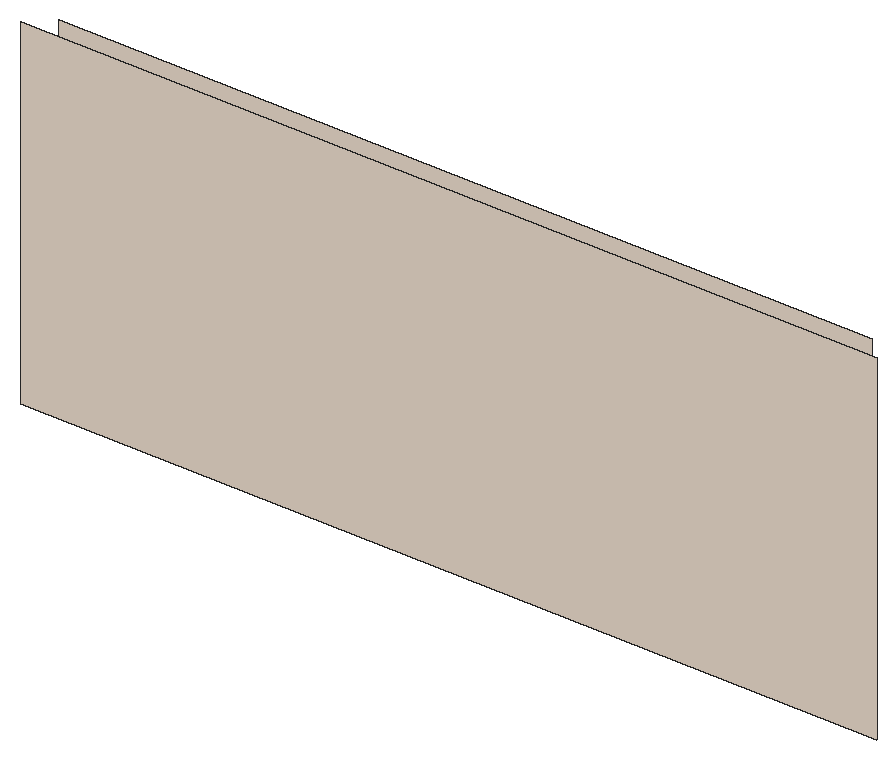
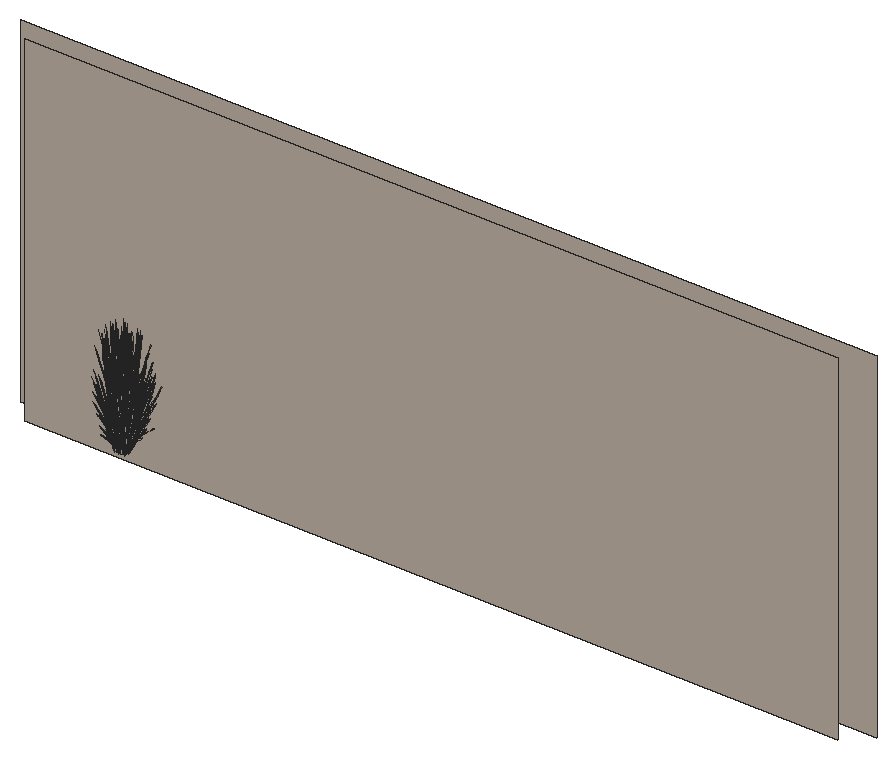
# SketchUp Ruby script. Lengths in inches.
U = 1.inch
M = Sketchup.active_model
def pt(a) = Geom::Point3d.new(a.map { |v| v * U })
def face(e, loops, mat)
  f = e.add_face(loops[0].map { |a| pt(a) })
  loops[1..].each { |l| e.add_face(l.map { |a| pt(a) }).erase! }
  f.material = f.back_material = mat if mat
  f
end
# faces: each face lists its corners as indices into pts; further lists are holes
def faces(e, pts, list, mat = nil) = list.each { |f| face(e, (f[0].is_a?(Array) ? f : [f]).map { |l| l.map { |i| pts[i] } }, mat) }
# xy, xz, yz: faces in a plane at the given z, y or x. An outline is a flat list of corners, or four numbers for a rectangle; further outlines are holes
def ring(l) = l.size == 4 ? [[l[0], l[1]], [l[2], l[1]], [l[2], l[3]], [l[0], l[3]]] : l.each_slice(2).to_a
def flat(e, list, mat, &to3) = list.each { |f| face(e, (f[0].is_a?(Array) ? f : [f]).map { |l| ring(l).map { |u, v| to3.(u, v) } }, mat) }
def xy(e, z, list, mat = nil) = flat(e, list, mat) { |x, y| [x, y, z] }
def xz(e, y, list, mat = nil) = flat(e, list, mat) { |x, z| [x, y, z] }
def yz(e, x, list, mat = nil) = flat(e, list, mat) { |y, z| [x, y, z] }
def lines(e, pts, list) = list.each { |a, b| e.add_line(pt(pts[a]), pt(pts[b])) }
# prism: a flat outline (further loops are holes) pulled along v
def prism(e, loops, v, mat = nil)
  f = face(e, loops, mat); d = Geom::Vector3d.new(v.map { |x| x * U })
  f.pushpull(f.normal.samedirection?(d) ? d.length : -d.length)
end
def box(e, o, s, mat = nil) = prism(e, [[o, [o[0] + s[0], o[1], o[2]], [o[0] + s[0], o[1] + s[1], o[2]], [o[0], o[1] + s[1], o[2]]]], [0, 0, s[2]], mat)
def at(x, y, z, deg = 0) = Geom::Transformation.translation(pt([x, y, z])) * Geom::Transformation.rotation(ORIGIN, Z_AXIS, deg.degrees)
def axes(o, x, y, z) = Geom::Transformation.new([*x, 0, *y, 0, *z, 0, *pt(o).to_a, 1])
def part(name) = M.definitions.add(name)
# library, detail: a bought-in or finely detailed component or shape, given as its bounding box
def library(name, o, s) = part(name).tap { |d| box(d.entities, o, s) }
def detail(e, o, s) = box(e.add_group.entities, o, s)
def put(e, d, t, mat = nil) = e.add_instance(d, t).tap { |i| i.material = mat if mat }
def group(e, t, mat = nil) = e.add_group.tap { |g| g.transformation = t; g.material = mat if mat }.entities
root = M.entities
M.materials.add("C01_Vanilla_Cream").color = [244, 228, 212]
M.materials.add("LightPink_Translucent").color = [144, 107, 117]
M.materials["LightPink_Translucent"].alpha = 0.75
c1 = part("blade")
p = [[2.15,0.21,22],[0,0.17,0],[0.09,0.45,0],[2.18,0.31,22],[2.29,0.31,22],[0.38,0.45,0],
  [2.48,0.24,33],[2.49,0.24,33],[2.48,0.22,33]]
faces(c1.entities,p,[[0,1,2,3],[4,5,2,3],[6,3,4,7],[8,0,3,6]])
c2 = part("seeds")
p = [[0.3,-0.1,1.38],[-0.01,-0.03,1.59],[-0.01,-0.03,0.03],[0.14,-0.07,-0.07],[0.29,-0.03,3],[0.15,0.01,3.11]]
faces(c2.entities,p,[[0,1,2,3],[1,0,4,5]],"LightPink_Translucent")
c3 = part("blade with seeds")
put(c3.entities,c1,at(0,0,0))
put(c3.entities,c2,axes([2.4,0.25,30.99],[1.5799,-0.05474,1.17369],[-0.12525,1.92788,0.29478],[-0.07173,-0.02425,1.56792]))
xz(root,0,[[0,300,360,444]],"C01_Vanilla_Cream")
xz(root,9,[[9,300,351,444]],"C01_Vanilla_Cream")
put(root,c3,axes([296.26,22.27,314.91],[0.23093,-0.01116,1.28532],[-0.15319,0.4836,0.10393],[-0.32909,-0.02991,0.54946]))
put(root,c3,axes([296.35,23.12,314.91],[0.19317,-0.10421,1.28532],[0.16263,0.48153,0.10393],[-0.30326,0.10883,0.54946]))
put(root,c3,axes([295.75,23.9375,313.94],[0.19348,0.04044,1.07251],[0.1247,0.41309,-0.23066],[-0.26282,0.07733,0.45856]))
put(root,c3,axes([297.46,22.62,314.51],[0.15825,-0.07127,1.32798],[0.05457,0.4976,0.10393],[-0.34278,0.06603,0.47463]))
put(root,c3,axes([295.76,22.95,315.54],[-0.09091,0.06396,1.31208],[0.00773,0.46734,-0.2075],[-0.20839,0.06078,0.10523]))
put(root,c3,axes([296.95,21.82,315.74],[-0.55654,-0.01186,-0.53284],[0.03738,-0.49951,0.0643],[-0.23578,-0.05271,0.75375]))
put(root,c3,axes([296.5,21.94,313.94],[0.1087,0.13716,1.07251],[-0.25048,0.37284,-0.23066],[-0.25719,-0.08912,0.45856]))
put(root,c3,axes([296.05,22.68,315.39],[-0.46269,-0.13744,-0.2656],[0.13495,-0.40096,0.3429],[-0.18628,0.03677,0.65611]))
put(root,c3,axes([296.69,21.49,314.91],[0.2068,0.08488,1.28532],[-0.42797,0.35609,0.10393],[-0.26673,-0.16064,0.54946]))
put(root,c3,axes([294.75,23.42,315.53],[0.07105,0.01321,1.33037],[0.2198,0.43529,-0.12571],[-0.14545,0.11425,0.23543]))
put(root,c3,axes([296.37,22.89,315.51],[-0.15083,0.44814,-0.38324],[-0.51712,-0.15361,-0.29685],[-0.2082,0.04109,0.7333]))
put(root,c3,axes([296.76,21.92,315.51],[-0.40426,0.32635,-0.38324],[-0.35404,-0.34474,-0.29685],[-0.2054,-0.04965,0.7333]))
put(root,c3,axes([296.11,22.86,313.12],[0.01412,0.07764,1.32257],[-0.28464,0.40547,-0.20205],[-0.20218,-0.02044,0.22528]))
put(root,c3,axes([296.19,21,315.53],[0.04127,0.04917,1.33037],[-0.19898,0.44196,-0.12571],[-0.20151,0.0032,0.23543]))
put(root,c3,axes([295.35,24.8,314.07],[0.23202,-0.22328,0.86145],[0.09155,0.35348,0.63294],[-0.16768,0.06329,0.18974]))
put(root,c3,axes([296.65,20.71,315.54],[-0.11979,-0.00348,1.31208],[-0.38137,0.34775,-0.2075],[-0.20349,-0.07106,0.10523]))
put(root,c3,axes([296.16,22.63,315.55],[0.15729,-0.44921,0.36002],[0.51712,0.15361,0.29685],[-0.20336,0.027,0.74497]))
put(root,c3,axes([296.35,22.5,315.78],[0.28012,0.44611,-0.0912],[-0.49717,0.21923,-0.50621],[-0.20951,0.05886,0.76918]))
put(root,c3,axes([296.98,21.58,315.78],[-0.02981,0.50103,-0.0912],[-0.56442,-0.01369,-0.50621],[-0.21738,-0.0348,0.76918]))
put(root,c3,axes([296.61,21.61,315.39],[-0.31678,-0.30846,-0.2656],[0.36171,-0.29199,0.3429],[-0.18378,-0.04443,0.65611]))
put(root,c3,axes([296.12,22.51,315.55],[-0.20448,-0.33592,0.04823],[0.37288,-0.16442,0.37966],[-0.16437,0.03244,0.57892]))
put(root,c3,axes([297.06,23.44,314.91],[0.13906,-0.15138,1.28532],[0.35111,0.40859,0.10393],[-0.24082,0.18608,0.54946]))
put(root,c3,axes([296.22,23.84,315.39],[-0.48462,0.07041,-0.2656],[-0.12797,-0.4025,0.3429],[-0.13888,0.10811,0.65611]))
put(root,c3,axes([295.96,25.03,313.12],[0.07468,0.04922,1.32257],[0.12663,0.45605,-0.20205],[-0.16551,0.09725,0.22528]))
put(root,c3,axes([295.85,22.35,314.07],[0.35544,-0.03525,0.86145],[-0.22547,0.31061,0.63294],[-0.17565,-0.04659,0.18974]))
put(root,c3,axes([296.29,23.75,315.55],[-0.13808,-0.45342,0.36002],[0.54163,-0.07869,0.29685],[-0.15963,0.10664,0.74497]))
put(root,c3,axes([296.57,21.5,315.82],[0.45978,-0.36358,0.40322],[0.39653,0.38611,0.33247],[-0.21571,-0.06707,0.83437]))
put(root,c3,axes([296.18,23.66,315.55],[-0.3822,-0.20719,0.04823],[0.22252,-0.29505,0.37966],[-0.12254,0.09539,0.57892]))
put(root,c3,axes([296.96,23.82,314.91],[0.10366,-0.16934,1.28532],[0.43488,0.35044,0.10393],[-0.19618,0.21841,0.54946]))
put(root,c3,axes([296.54,22.64,315.79],[0.46269,0.13744,0.2656],[-0.13495,0.40096,-0.3429],[-0.18628,0.03677,0.65611]))
put(root,c3,axes([296.62,23.89,315.51],[0.14302,0.44985,-0.38324],[-0.54163,0.07869,-0.29685],[-0.15522,0.12083,0.7333]))
put(root,c3,axes([296.78,21.49,315.55],[0.02803,-0.37463,0.04823],[0.42332,0.01027,0.37966],[-0.16216,-0.0392,0.57892]))
put(root,c3,axes([295.78,24.69,315.54],[-0.01384,0.09749,1.31208],[0.39274,0.33916,-0.2075],[-0.10282,0.16039,0.10523]))
put(root,c3,axes([297.97,23.5625,313.54],[-0.57914,-0.08077,-0.46765],[0.12221,-0.49823,-0.12274],[-0.17283,-0.06037,1.03225]))
put(root,c3,axes([298.08,20.85,316.07],[-0.37157,0.4723,-0.10215],[-0.5381,-0.2721,-0.56695],[-0.18705,-0.13344,0.86148]))
put(root,c3,axes([297.0625,21.77,315.79],[0.31678,0.30846,0.2656],[-0.36171,0.29199,-0.3429],[-0.18378,-0.04443,0.65611]))
put(root,c3,axes([297.92,21.23,315.74],[-0.47473,-0.23813,-0.53284],[0.33738,-0.41728,0.0643],[-0.172,-0.14218,0.75375]))
put(root,c3,axes([297.69,21.24,315.51],[-0.54938,0.11711,-0.38324],[-0.0961,-0.44351,-0.29685],[-0.14756,-0.1271,0.7333]))
put(root,c3,axes([297.21,24.51,313.51],[-0.52105,-0.24633,-0.37238],[0.31144,-0.44171,0],[-0.11867,-0.0561,1.18128]))
put(root,c3,axes([296.98,20.84,313.12],[-0.05393,0.0649,1.32257],[-0.545,0.13993,-0.20205],[-0.13166,-0.12729,0.22528]))
put(root,c3,axes([296.37,23.5625,315.78],[0.515,0.27165,-0.0912],[-0.2967,0.3934,-0.50621],[-0.1455,0.13675,0.76918]))
put(root,c3,axes([297.53,24.8,313.78],[-0.34808,0.49367,0],[-0.58235,-0.27531,-0.38706],[-0.13264,-0.0627,1.22783]))
put(root,c3,axes([295.52,24.74,316.23],[0.49129,0.13151,-0.04866],[-0.15113,0.40475,-0.22062],[-0.08035,0.06145,0.72768]))
put(root,c3,axes([296.62,23.6,315.79],[0.48462,-0.07041,0.2656],[0.12797,0.4025,-0.3429],[-0.13888,0.10811,0.65611]))
put(root,c3,axes([296.9,25.52,313.94],[0.17569,-0.07772,1.07251],[0.43377,0.23434,-0.23066],[-0.12911,0.20277,0.45856]))
put(root,c3,axes([296.65,21.09,313.6],[-0.1606,0.40228,-0.02919],[-0.4943,-0.12375,-0.13237],[-0.07505,-0.0658,0.43661]))
put(root,c3,axes([297.93,19.72,315.53],[-0.01039,0.05905,1.33037],[-0.51226,0.21431,-0.12571],[-0.15074,-0.10955,0.23543]))
put(root,c3,axes([297.38,20.58,313.94],[-0.03371,0.16116,1.07251],[-0.49286,0.13491,-0.23066],[-0.11521,-0.20831,0.45856]))
put(root,c3,axes([297.55,21,314.91],[0.12726,0.15818,1.28532],[-0.58807,0.13317,0.10393],[-0.13291,-0.24832,0.54946]))
put(root,c3,axes([298.63,23.64,314],[-0.56211,0.32708,-0.21822],[-0.3738,-0.46216,-0.37502],[-0.13869,-0.04694,1.19781]))
put(root,c3,axes([297.08,24.67,315.55],[-0.39645,-0.33614,0.36002],[0.42102,-0.2899,0.29685],[-0.07313,0.15771,0.74497]))
put(root,c3,axes([297.75,20.91,315.39],[-0.08599,-0.39682,-0.2656],[0.49155,-0.10478,0.3429],[-0.13203,-0.11372,0.65611]))
put(root,c3,axes([296.38,22.92,313.78],[-0.69617,0,0],[0,-0.55062,-0.38706],[0,-0.12541,1.22783]))
put(root,c3,axes([297.36,24.32,313.52],[-0.13078,-0.42928,-0.23233],[0.51941,-0.1219,0.23233],[-0.10471,-0.0495,1.0423]))
put(root,c3,axes([296.93,24.64,315.55],[-0.45752,-0.02296,0.04823],[0.01254,-0.34663,0.37966],[-0.04787,0.13278,0.57892]))
put(root,c3,axes([297.08,24.77,315.39],[-0.3767,0.25939,-0.2656],[-0.3566,-0.29618,0.3429],[-0.05426,0.15048,0.65611]))
put(root,c3,axes([299,23.99,313.54],[-0.375,0.3703,-0.46765],[-0.46584,-0.33578,-0.12274],[-0.15027,0.09237,1.03225]))
put(root,c3,axes([298.04,21.24,315.79],[0.08599,0.39682,0.2656],[-0.49155,0.10478,-0.3429],[-0.13203,-0.11372,0.65611]))
put(root,c3,axes([295.73,25.69,315.53],[0.06316,-0.02974,1.33037],[0.52204,0.19785,-0.12571],[-0.01227,0.16473,0.23543]))
put(root,c3,axes([296.92,22.78,313.75],[-0.51786,0.4142,0.23067],[-0.51817,-0.40984,-0.27369],[-0.01808,-0.11762,1.23664]))
put(root,c3,axes([299.05,23.92,314.49],[0.48111,0.19866,1.13446],[-0.47133,0.42798,0.44862],[-0.21112,-0.25366,0.95105]))
put(root,c3,axes([297.21,20.32,314.07],[0.29042,0.17147,0.86145],[-0.42295,0.10307,0.63294],[-0.0905,-0.13178,0.18974]))
put(root,c3,axes([299.26,23.79,313.85],[-0.54364,-0.39653,-0.18894],[0.45745,-0.44527,0.41347],[-0.14639,0.04639,1.26162]))
put(root,c3,axes([298.27,23.4,313.66],[-0.33445,-0.41351,-0.33554],[0.50659,-0.29119,0.16149],[-0.10823,-0.05117,1.07733]))
put(root,c3,axes([297.33,24.5,316],[-0.01449,0.45571,-0.59145],[-0.61002,-0.03061,0.07138],[-0.06438,0.19306,0.83667]))
put(root,c3,axes([297.32,25.78,314.07],[-0.01441,-0.29294,0.86145],[0.36003,0.20894,0.63294],[-0.07081,0.13963,0.18974]))
put(root,c3,axes([297.82,20.77,315.82],[0.62019,-0.12663,0.40322],[0.10763,0.49673,0.33247],[-0.14586,-0.1464,0.83437]))
put(root,c3,axes([298.99,23.7,313.66],[-0.60457,0.03041,-0.33554],[-0.05467,-0.50484,0.16149],[-0.10823,0.05117,1.07733]))
put(root,c3,axes([297.96,20.88,315.55],[0.25304,-0.31296,0.04823],[0.36033,0.18221,0.37966],[-0.11649,-0.10034,0.57892]))
put(root,c3,axes([297.83,24.55,313.86],[0.52105,0.24633,0.37238],[-0.31144,0.44171,0],[-0.11867,-0.0561,1.18128]))
put(root,c3,axes([297.12,25.14,314.52],[0.01223,-0.25433,1.15759],[0.55017,0.13434,0.15997],[-0.04767,0.27105,0.54661]))
put(root,c3,axes([298.32,23.64,313.83],[0.14756,-0.58378,-0.17572],[0.69966,0.10176,0.38453],[-0.12225,-0.08062,1.1733]))
put(root,c3,axes([298.58,23.78,313.96],[-0.1074,0.43968,0.1086],[-0.52474,-0.07632,-0.3101],[-0.0955,-0.04515,0.95058]))
put(root,c3,axes([298.52,19.95,315.54],[-0.08515,-0.06907,1.31208],[-0.56828,0.04379,-0.2075],[-0.0907,-0.16522,0.10523]))
put(root,c3,axes([299.62,25,313.51],[-0.52105,0.24633,-0.37238],[-0.31144,-0.44171,0],[-0.11867,0.0561,1.18128]))
put(root,c3,axes([296.54,22.55,313.51],[0,-0.49266,-0.37238],[0.62289,0,0],[0,-0.11221,1.18128]))
put(root,c3,axes([296.8,23.01,313.86],[0,0.49266,0.37238],[-0.62289,0,0],[0,-0.11221,1.18128]))
put(root,c3,axes([299.66,24.87,313.64],[-0.34375,-0.4954,-0.03857],[0.58235,-0.27531,0.38706],[-0.1435,0.04717,1.22723]))
put(root,c3,axes([297.45,24.65,315.75],[0.39855,0.33102,-0.4254],[-0.42102,0.2899,-0.32951],[-0.06064,0.16819,0.81396]))
put(root,c3,axes([299.5,24.81,313.52],[-0.51941,-0.1219,-0.23233],[0.13078,-0.42928,0.23233],[-0.10471,0.0495,1.0423]))
put(root,c3,axes([297.27,24.4,315.79],[0.3767,-0.25939,0.2656],[0.3566,0.29618,-0.3429],[-0.05426,0.15048,0.65611]))
put(root,c3,axes([298.16,23.12,314],[-0.62699,-0.23507,-0.21822],[0.3019,-0.49615,-0.37502],[-0.0197,-0.12182,1.19781]))
put(root,c3,axes([299.8,22.97,314.13],[-0.01521,-0.46386,1.05954],[0.68831,0.12024,0.44862],[-0.1628,0.25382,1.00012]))
put(root,c3,axes([297.03,24.47,316.05],[0.61188,0.02441,-0.10123],[-0.01672,0.46217,-0.56189],[-0.0425,0.178,0.85379]))
put(root,c3,axes([297.02,25.15,314.12],[0.50577,-0.08724,0.04881],[0.11627,0.35148,-0.64728],[-0.03206,0.17792,0.5802]))
put(root,c3,axes([299.41,23.57,314],[0.06488,0.56215,-0.21822],[-0.6757,0.03399,-0.37502],[-0.11898,0.07488,1.19781]))
put(root,c3,axes([297.88,22.62,313.57],[-0.22864,-0.5052,-0.52377],[0.65862,-0.18195,-0.13747],[-0.02527,-0.17107,1.15612]))
put(root,c3,axes([299.38,21.02,315.78],[-0.54481,0.22937,-0.0912],[-0.26773,-0.4071,-0.50621],[-0.07188,-0.17155,0.76918]))
put(root,c3,axes([298.91,21.04,315.51],[-0.54728,-0.1235,-0.38324],[0.18759,-0.42344,-0.29685],[-0.05018,-0.17048,0.7333]))
put(root,c3,axes([297.9,24.17,314.91],[-0.01363,-0.18909,1.28532],[0.5906,0.12544,0.10393],[-0.03653,0.26947,0.54946]))
put(root,c3,axes([296.8,22.5625,313.52],[0.38863,-0.30738,-0.23233],[0.38863,0.30738,0.23233],[0,-0.09901,1.0423]))
put(root,c3,axes([298.56,20.57,313.6],[-0.38473,0.28263,-0.02919],[-0.35252,-0.30954,-0.13237],[-0.02482,-0.08771,0.43661]))
put(root,c3,axes([298.4,23.36,313.77],[0.70367,0.1038,0.34316],[-0.1432,0.58624,0.13466],[-0.10283,-0.05661,1.19142]))
put(root,c3,axes([298.22,23.25,314.04],[-0.27012,0.44393,0.33554],[-0.56127,-0.21365,-0.16149],[0,-0.10233,1.07733]))
put(root,c3,axes([299.11,21.12,315.74],[-0.26572,-0.40059,-0.53284],[0.54698,-0.22325,0.0643],[-0.06214,-0.19355,0.75375]))
put(root,c3,axes([298.03,24.3,313.86],[0.59825,-0.13076,0.13232],[0.14773,0.48663,0.26315],[-0.05336,-0.0709,1.20305]))
put(root,c3,axes([298.8,24.375,313.65],[-0.56127,-0.22118,0],[0.27012,-0.45959,0],[0,0,1.2203]))
put(root,c3,axes([299.22,21.17,315.79],[-0.16784,0.37886,0.2656],[-0.48968,-0.1105,-0.3429],[-0.0449,-0.15254,0.65611]))
put(root,c3,axes([300.09,24.93,313.78],[0.34808,0.49367,0],[-0.58235,0.27531,-0.38706],[-0.13264,0.0627,1.22783]))
put(root,c3,axes([298.32,25.14,315.8],[-0.54859,-0.1288,0.39962],[0.18759,-0.42344,0.32951],[0.03297,0.16652,0.82692]))
put(root,c3,axes([298.18,25.17,315.55],[-0.41024,0.16744,0.04823],[-0.2008,-0.30532,0.37966],[0.03962,0.13459,0.57892]))
put(root,c3,axes([299.81,24.32,313.86],[0.16083,-0.48962,0.13232],[0.58854,0.13856,0.26315],[-0.10167,0.00238,1.20305]))
put(root,c3,axes([299.53,23.67,313.96],[0.41131,0.296,0.1086],[-0.34309,0.33395,-0.3101],[-0.0955,0.04515,0.95058]))
put(root,c3,axes([299.39,23.31,313.72],[-0.51786,-0.42404,-0.04598],[0.51817,-0.4243,0],[-0.01808,-0.01481,1.31678]))
put(root,c3,axes([299.52,23.46,314.04],[0.60457,-0.03041,0.33554],[0.05467,0.50484,-0.16149],[-0.10823,0.05117,1.07733]))
put(root,c3,axes([299.67,24.62,313.75],[0.697,0.16013,0.23067],[-0.17437,0.57237,-0.27369],[-0.11536,0.07164,1.23664]))
put(root,c3,axes([298.65,20.23,313.12],[-0.09338,0.01775,1.32257],[-0.51641,-0.1998,-0.20205],[0.00867,-0.16666,0.22528]))
put(root,c3,axes([299.97,24.59,313.86],[0.52105,-0.24633,0.37238],[0.31144,0.44171,0],[-0.11867,0.0561,1.18128]))
put(root,c3,axes([299.16,20.78,315.39],[0.16784,-0.37886,-0.2656],[0.48968,0.1105,0.3429],[-0.0449,-0.15254,0.65611]))
put(root,c3,axes([298.34,22.82,313.77],[0.24206,0.5509,0.34316],[-0.69162,0.19157,0.13466],[0.00845,-0.10123,1.19142]))
put(root,c3,axes([298.23,22.75,313.66],[0.27012,-0.44393,-0.33554],[0.56127,0.21365,0.16149],[0,-0.10233,1.07733]))
put(root,c3,axes([298.92,24.18,313.65],[-0.18165,-0.42474,0],[0.51872,-0.14874,0],[0,0,1.15778]))
put(root,c3,axes([298.26,25.08,313.12],[0.0901,-0.02681,1.32257],[0.54199,0.14755,-0.20205],[0.01585,0.1663,0.22528]))
put(root,c3,axes([298.38,25.23,315.39],[-0.16784,0.37886,-0.2656],[-0.48968,-0.1105,0.3429],[0.0449,0.15254,0.65611]))
put(root,c3,axes([299.66,23.35,313.66],[-0.27012,0.44393,-0.33554],[-0.56127,-0.21365,0.16149],[0,0.10233,1.07733]))
put(root,c3,axes([299.37,20.83,315.55],[0.41024,-0.16744,0.04823],[0.2008,0.30532,0.37966],[-0.03962,-0.13459,0.57892]))
put(root,c3,axes([298.04,25.9,315.54],[0.07057,0.07933,1.31208],[0.56952,0.03117,-0.2075],[0.05727,0.17496,0.10523]))
put(root,c3,axes([300.72,23.07,313.86],[-0.43742,-0.35886,0.13232],[0.44081,-0.34807,0.26315],[-0.04831,0.07329,1.20305]))
put(root,c3,axes([299.21,22.87,313.65],[0,-0.57005,0],[0.69617,0,0],[0,0,1.34592]))
put(root,c3,axes([299.22,20.86,315.55],[0.54859,0.1288,0.36002],[-0.18759,0.42344,0.29685],[-0.03297,-0.16652,0.74497]))
put(root,c3,axes([298.57,22.97,313.82],[0.6273,0.23878,0.18048],[-0.3019,0.49615,0.37502],[0,-0.11437,1.20407]))
put(root,c3,axes([299.5625,23.1,313.72],[0,0.56976,-0.04228],[-0.69617,0,0],[0,0.01791,1.34526]))
put(root,c3,axes([298.36,22.64,314.04],[-0.60457,0.03041,0.33554],[-0.05467,-0.50484,-0.16149],[0.10823,-0.05117,1.07733]))
put(root,c3,axes([298.33,24.83,315.79],[0.16784,-0.37886,0.2656],[0.48968,0.1105,-0.3429],[0.0449,0.15254,0.65611]))
put(root,c3,axes([298.08,21.77,313.86],[-0.16083,0.48962,0.13232],[-0.58854,-0.13856,0.26315],[0.10167,-0.00238,1.20305]))
put(root,c3,axes([299.23,24.2,313.72],[0.24206,0.56598,-0.04509],[-0.69162,0.19832,0],[0.00845,0.01976,1.2913]))
put(root,c3,axes([297.79,21.17,313.78],[-0.34808,-0.49367,0],[0.58235,-0.27531,-0.38706],[0.13264,-0.0627,1.22783]))
put(root,c3,axes([298.43,24.89,315.74],[0.26572,0.40059,-0.53284],[-0.54698,0.22325,0.0643],[0.06214,0.19355,0.75375]))
put(root,c3,axes([301.23,23.46,313.65],[-0.69582,-0.00394,-0.03732],[0,-0.55062,0.37457],[-0.02187,0.12535,1.18764]))
put(root,c3,axes([299.86,21.8,313.86],[-0.59825,0.13076,0.13232],[-0.14773,-0.48663,0.26315],[0.05336,0.0709,1.20305]))
put(root,c3,axes([299.25,19.98,314.07],[0.07142,0.28728,0.86145],[-0.3962,-0.15911,0.63294],[0.04263,-0.1471,0.18974]))
put(root,c3,axes([298.99,26.18,316.23],[0.38473,-0.28263,-0.04866],[0.35252,0.30954,-0.22062],[0.02482,0.08771,0.72768]))
put(root,c3,axes([298.88,22.51,313.77],[-0.46162,0.4471,0.34316],[-0.54842,-0.39467,0.13466],[0.11129,-0.04462,1.19142]))
put(root,c3,axes([299.67,23.21,313.66],[0.38863,0.31822,0],[-0.38863,0.31822,0],[0,0,1.2695]))
put(root,c3,axes([299.67,22.84,314.04],[0.27012,-0.44393,0.33554],[0.56127,0.21365,-0.16149],[0,0.10233,1.07733]))
put(root,c3,axes([299.43,24.38,313.65],[0.56127,0.22118,0],[-0.27012,0.45959,0],[0,0,1.31215]))
put(root,c3,axes([298.63,24.97,315.51],[0.54728,0.1235,-0.38324],[-0.18759,0.42344,-0.29685],[0.05018,0.17048,0.7333]))
put(root,c3,axes([298.16,24.99,315.78],[0.54481,-0.22937,-0.0912],[0.26773,0.4071,-0.50621],[0.07188,0.17155,0.76918]))
put(root,c3,axes([299.48,22.74,313.79],[-0.70367,-0.1038,0.36899],[0.1432,-0.58624,0.1448],[0.10283,0.05661,1.2811]))
put(root,c3,axes([300.95,20.44,315.53],[-0.05654,0.03763,1.33037],[-0.55396,-0.12696,-0.12571],[-0.02005,-0.16422,0.23543]))
put(root,c3,axes([300.51,21.53,315.78],[-0.61188,-0.02441,-0.0912],[0.01672,-0.46217,-0.50621],[0.0425,-0.178,0.76918]))
put(root,c3,axes([301.08,23.54,313.52],[-0.38863,0.30738,-0.23233],[-0.38863,-0.30738,0.23233],[0,0.09901,1.0423]))
put(root,c3,axes([299.97,23.48,313.57],[0.20414,0.45107,-0.51909],[-0.58805,0.16245,-0.13624],[0.02256,0.15274,1.1458]))
put(root,c3,axes([299.6875,23,313.65],[0.62289,0,0],[0,0.51004,0],[0,0,1.33805]))
put(root,c3,axes([300.27,21.6,315.79],[-0.3767,0.25939,0.2656],[-0.3566,-0.29618,-0.3429],[0.05426,-0.15048,0.65611]))
put(root,c3,axes([299.09,22.43,314.04],[-0.33445,-0.41351,0.33554],[0.50659,-0.29119,-0.16149],[0.10823,0.05117,1.07733]))
put(root,c3,axes([298.48,22.53,314],[-0.06488,-0.56215,-0.21822],[0.6757,-0.03399,-0.37502],[0.11898,-0.07488,1.19781]))
put(root,c3,axes([299.9,22.94,313.96],[0.51872,-0.14368,0.1086],[0.18165,0.41027,-0.3101],[0,0.09029,0.95058]))
put(root,c3,axes([300.1,21.36,315.51],[-0.39855,-0.33102,-0.38324],[0.42102,-0.2899,-0.29685],[0.06064,-0.16819,0.7333]))
put(root,c3,axes([299.72,22.98,314],[0.62699,0.23507,-0.21822],[-0.3019,0.49615,-0.37502],[0.0197,0.12182,1.19781]))
put(root,c3,axes([298.39,21.29,313.52],[0.51941,0.1219,-0.23233],[-0.13078,0.42928,0.23233],[0.10471,-0.0495,1.0423]))
put(root,c3,axes([299.83,20.77,313.94],[-0.15825,0.09972,1.07251],[-0.47395,-0.17454,-0.23066],[0.08785,-0.21706,0.45856]))
put(root,c3,axes([301.09,23.09,313.86],[0,-0.49266,0.37238],[0.62289,0,0],[0,0.11221,1.18128]))
put(root,c3,axes([301.35,23.55,313.51],[0,0.49266,-0.37238],[-0.62289,0,0],[0,0.11221,1.18128]))
put(root,c3,axes([299.6875,25.04,315.55],[-0.55374,0.11306,0.36002],[-0.0961,-0.44351,0.29685],[0.13023,0.13071,0.74497]))
put(root,c3,axes([298.27,21.09,313.51],[0.52105,-0.24633,-0.37238],[0.31144,0.44171,0],[0.11867,-0.0561,1.18128]))
put(root,c3,axes([299.58,25.125,315.55],[-0.25304,0.31296,0.04823],[-0.36033,-0.18221,0.37966],[0.11649,0.10034,0.57892]))
put(root,c3,axes([298.94,24.1,314.91],[-0.12726,-0.15818,1.28532],[0.58807,-0.13317,0.10393],[0.13291,0.24832,0.54946]))
put(root,c3,axes([299.3125,22.32,313.96],[0.1074,-0.43968,0.1086],[0.52474,0.07632,-0.3101],[0.0955,0.04515,0.95058]))
put(root,c3,axes([300.06,21.55,313.86],[-0.52105,-0.24633,0.37238],[0.31144,-0.44171,0],[0.11867,0.0561,1.18128]))
put(root,c3,axes([300.22,21.51,315.74],[0.01449,-0.45571,-0.53284],[0.61002,0.03061,0.0643],[0.06438,-0.19306,0.75375]))
put(root,c3,axes([299.6,24.125,313.64],[0.5845,-0.16716,-0.14398],[0.20539,0.48152,0.00006],[0.06452,-0.01848,1.30423]))
put(root,c3,axes([299.5,24.77,315.79],[-0.08599,-0.39682,0.2656],[0.49155,-0.10478,-0.3429],[0.13203,0.11372,0.65611]))
put(root,c3,axes([299.61,22.69,313.66],[0.33445,0.41351,-0.33554],[-0.50659,0.29119,0.16149],[0.10823,0.05117,1.07733]))
put(root,c3,axes([299.84,22.48,315.36],[-0.48108,-0.25598,1.03712],[0.50798,-0.39855,0.44749],[0.15521,0.24018,1.00248]))
put(root,c3,axes([300.47,21.23,315.39],[0.3767,-0.25939,-0.2656],[0.3566,0.29618,0.3429],[0.05426,-0.15048,0.65611]))
put(root,c3,axes([299.03,25.32,315.53],[0.00165,-0.05965,1.33037],[0.47711,-0.26315,-0.12571],[0.16572,0.09393,0.23543]))
put(root,c3,axes([300.62,21.37,315.55],[0.45752,0.02296,0.04823],[-0.01254,0.34663,0.37966],[0.04787,-0.13278,0.57892]))
put(root,c3,axes([300.5625,24.57,314.07],[-0.31347,-0.14166,0.86145],[0.40476,-0.14393,0.63294],[0.10917,0.12192,0.18974]))
put(root,c3,axes([299.45,24.42,313.94],[0.00982,-0.16331,1.07251],[0.4695,-0.18242,-0.23066],[0.14493,0.19547,0.45856]))
put(root,c3,axes([301.07,20.8,315.54],[-0.00537,-0.09805,1.31208],[-0.45391,-0.28338,-0.2075],[0.07018,-0.17178,0.10523]))
put(root,c3,axes([298.88,22.1,313.54],[0.375,-0.3703,-0.46765],[0.46584,0.33578,-0.12274],[0.15027,-0.09237,1.03225]))
put(root,c3,axes([300.47,21.33,315.55],[0.39645,0.33614,0.36002],[-0.42102,0.2899,0.29685],[0.07313,-0.15771,0.74497]))
put(root,c3,axes([300.53,21.77,313.52],[0.13078,0.42928,-0.23233],[-0.51941,0.1219,0.23233],[0.10471,0.0495,1.0423]))
put(root,c3,axes([301.51,23.17,313.78],[0.69617,0,0],[0,0.55062,-0.38706],[0,0.12541,1.22783]))
put(root,c3,axes([299.26,22.46,314],[0.56211,-0.32708,-0.21822],[0.3738,0.46216,-0.37502],[0.13869,0.04694,1.19781]))
put(root,c3,axes([300.61,25.21,314],[-0.35702,-0.01545,0.78795],[0.23577,-0.32816,0.43504],[0.14104,0.11659,0.61808]))
put(root,c3,axes([300.93,22.4,315.79],[-0.48462,0.07041,0.2656],[-0.12797,-0.4025,-0.3429],[0.13888,-0.10811,0.65611]))
put(root,c3,axes([299.53,21.28,314.91],[-0.10366,0.16934,1.28532],[-0.43488,-0.35044,0.10393],[0.19618,-0.21841,0.54946]))
put(root,c3,axes([299.46,24.97,315.78],[0.33176,-0.4217,-0.0912],[0.48044,0.24295,-0.50621],[0.16701,0.11914,0.76918]))
put(root,c3,axes([297.84,22.17,313.2],[-0.548,0.19724,0.96696],[-0.17442,-0.56594,0.37572],[0.3365,0.00941,1.09981]))
put(root,c3,axes([301.18,22.44,315.78],[-0.515,-0.27165,-0.0912],[0.2967,-0.3934,-0.50621],[0.1455,-0.13675,0.76918]))
put(root,c3,axes([299.85,24.76,315.51],[0.54938,-0.11711,-0.38324],[0.0961,0.44351,-0.29685],[0.14756,0.1271,0.7333]))
put(root,c3,axes([300.36,21.29,313.78],[0.34808,-0.49367,0],[0.58235,0.27531,-0.38706],[0.13264,0.0627,1.22783]))
